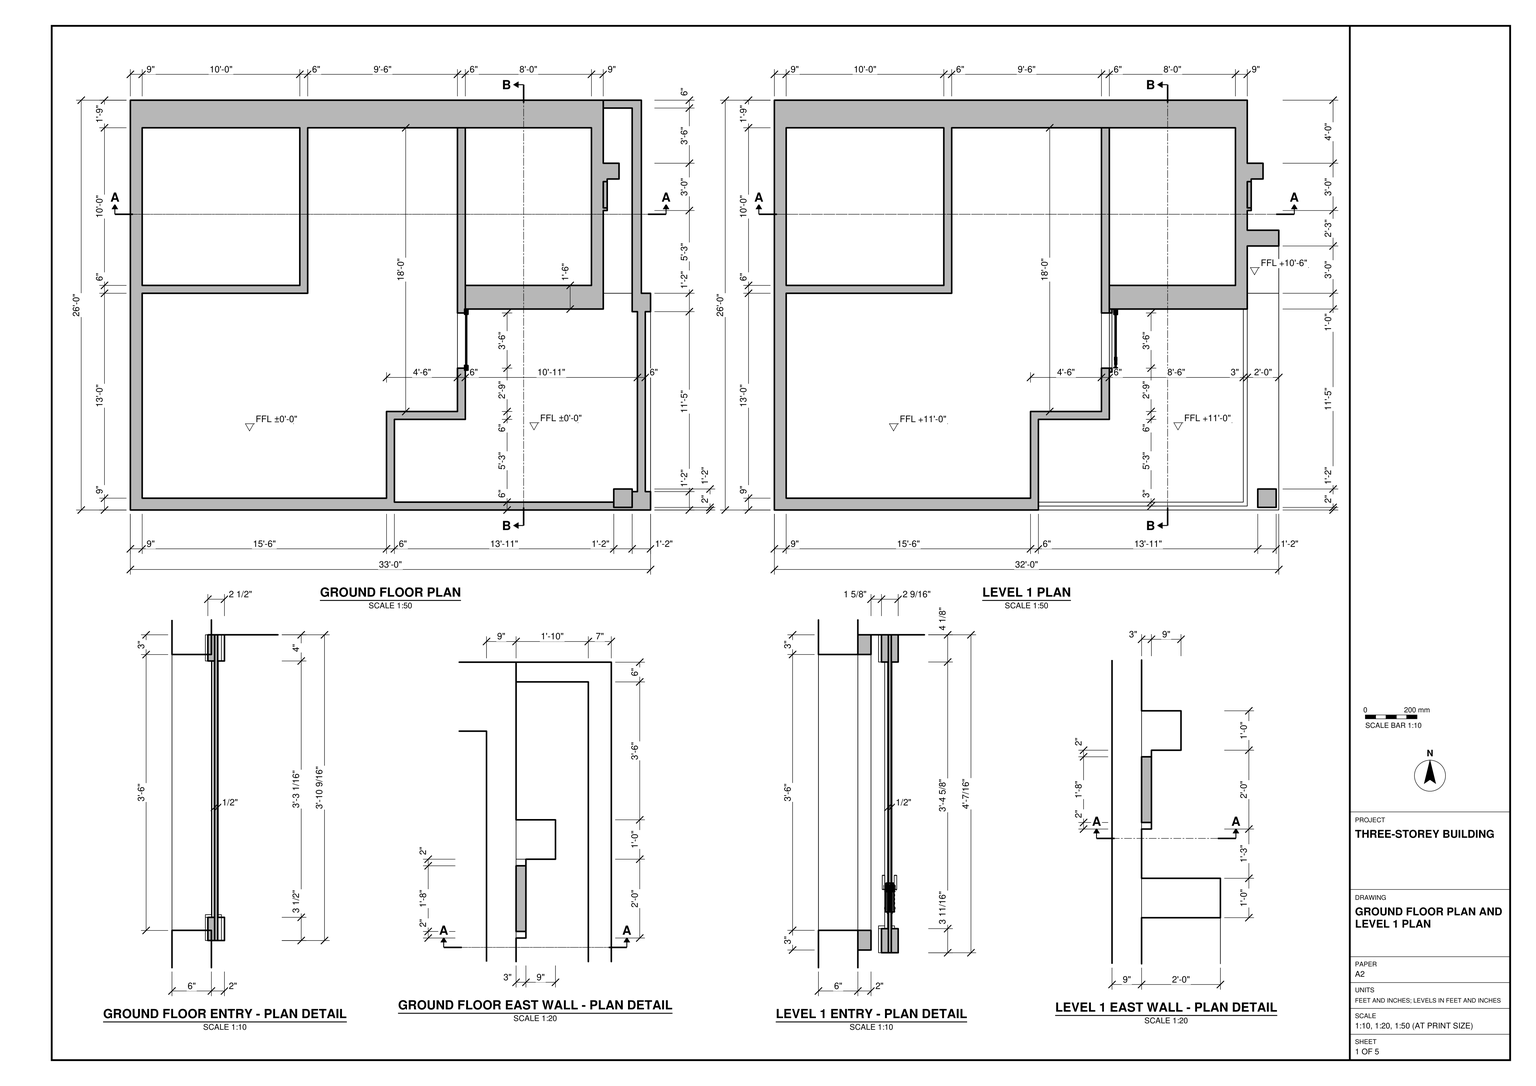
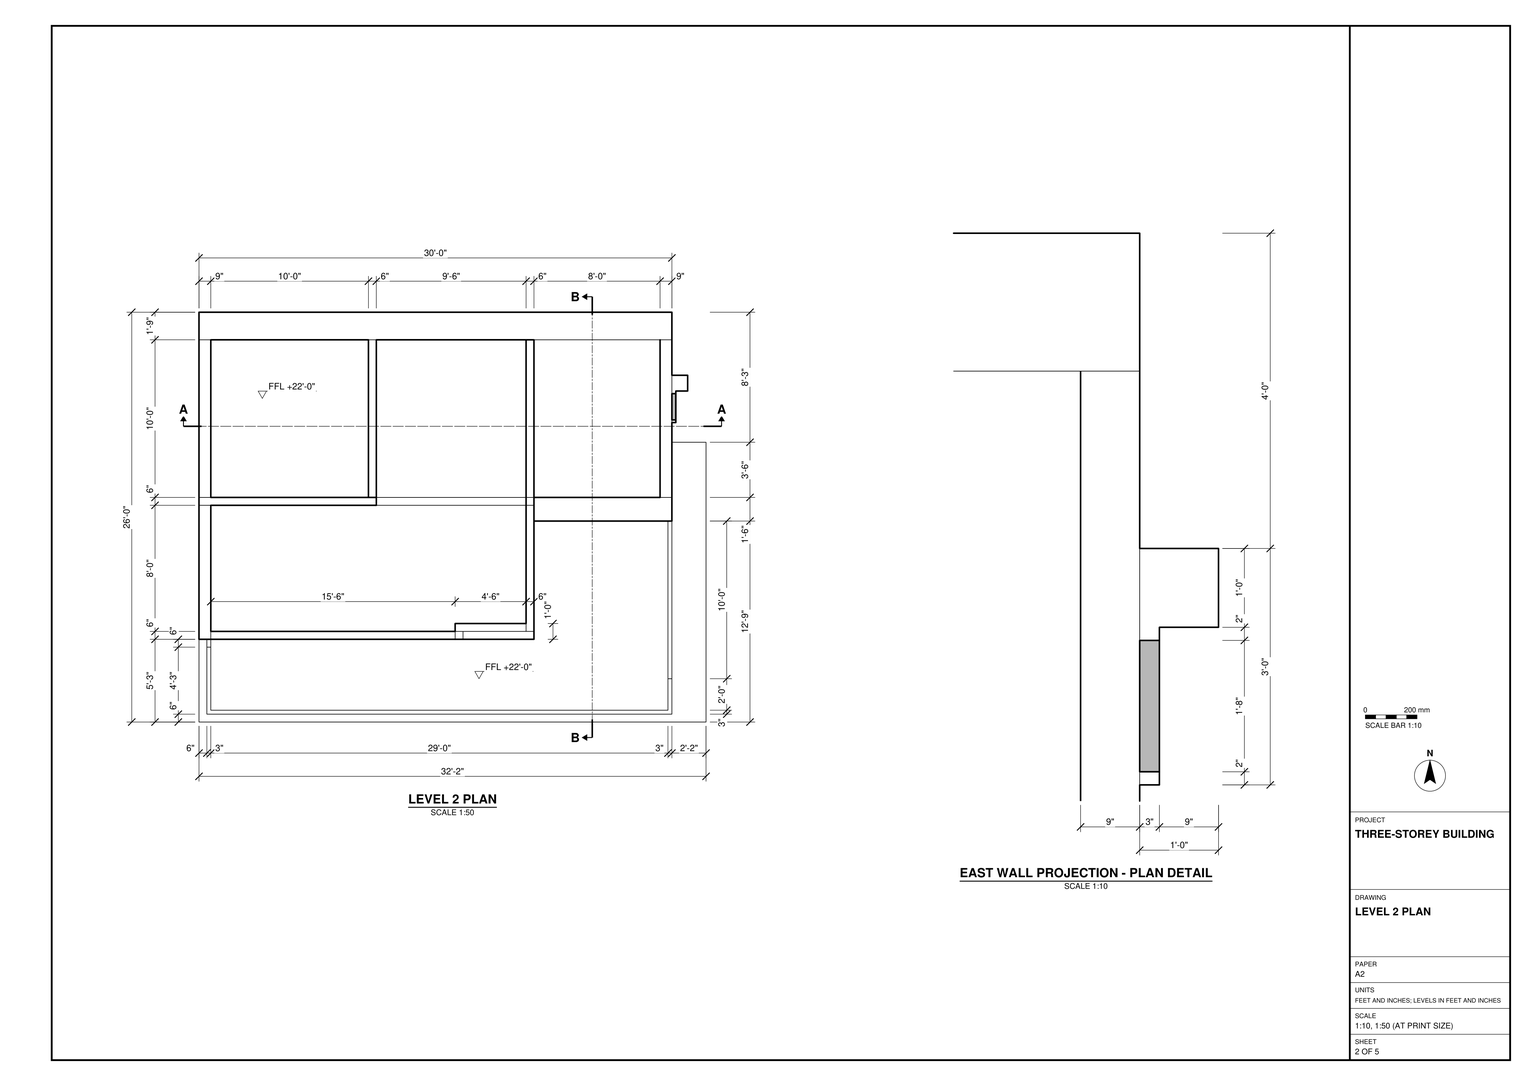
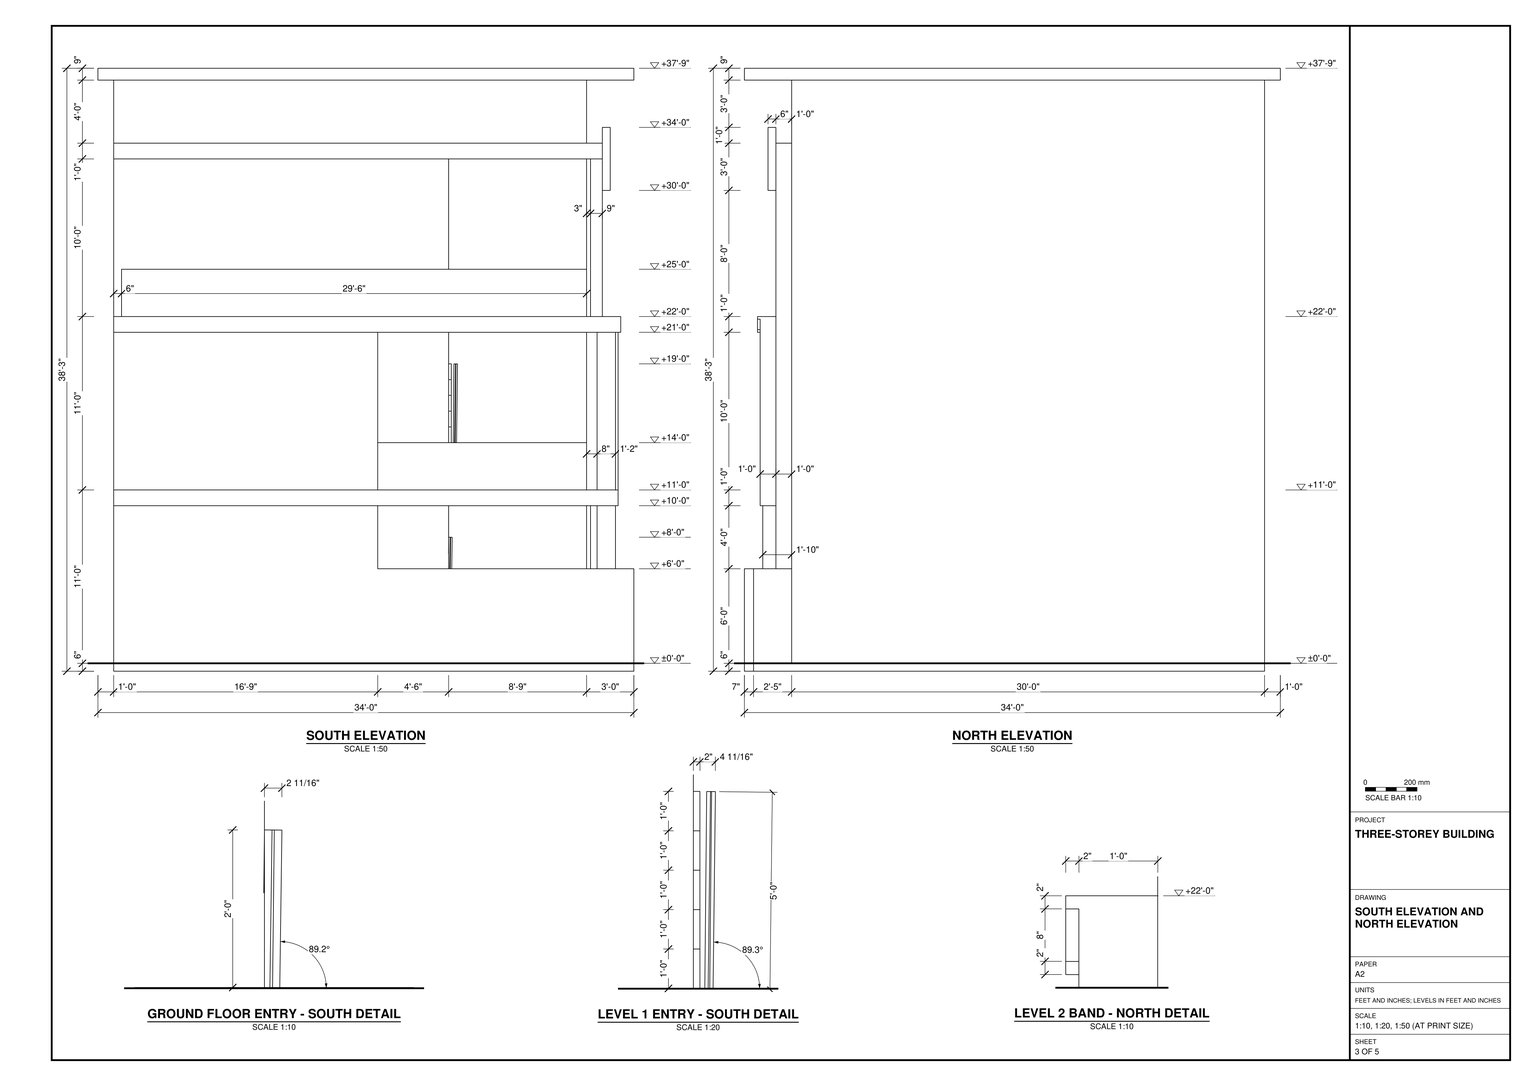
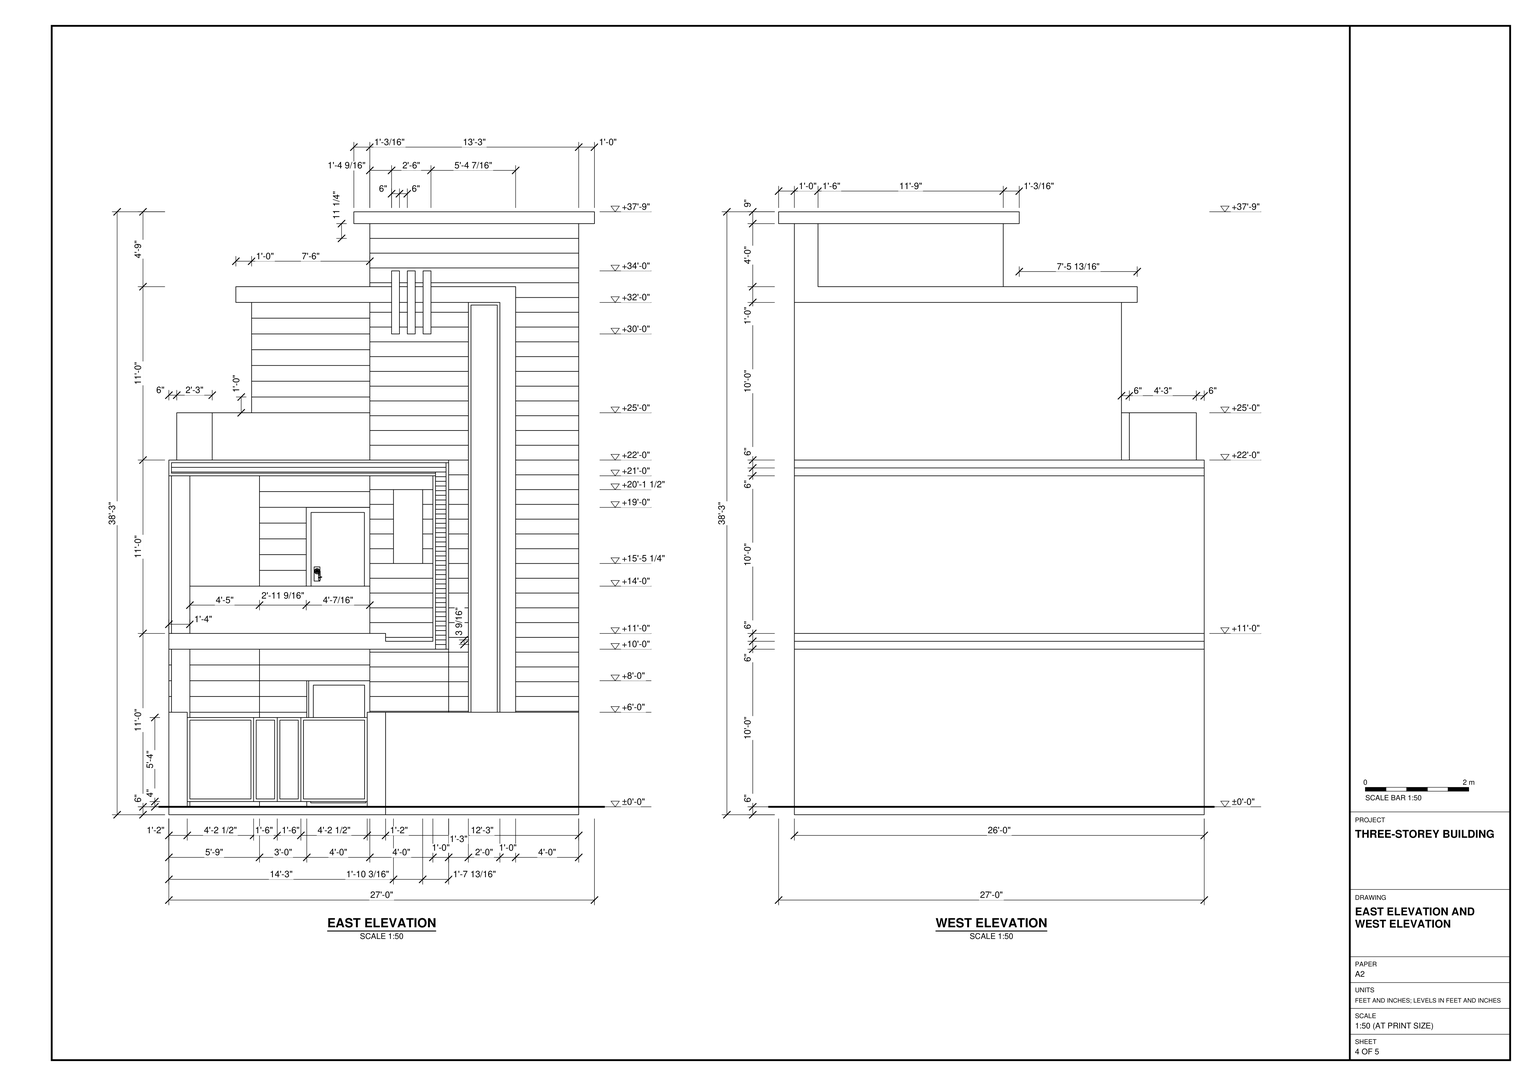
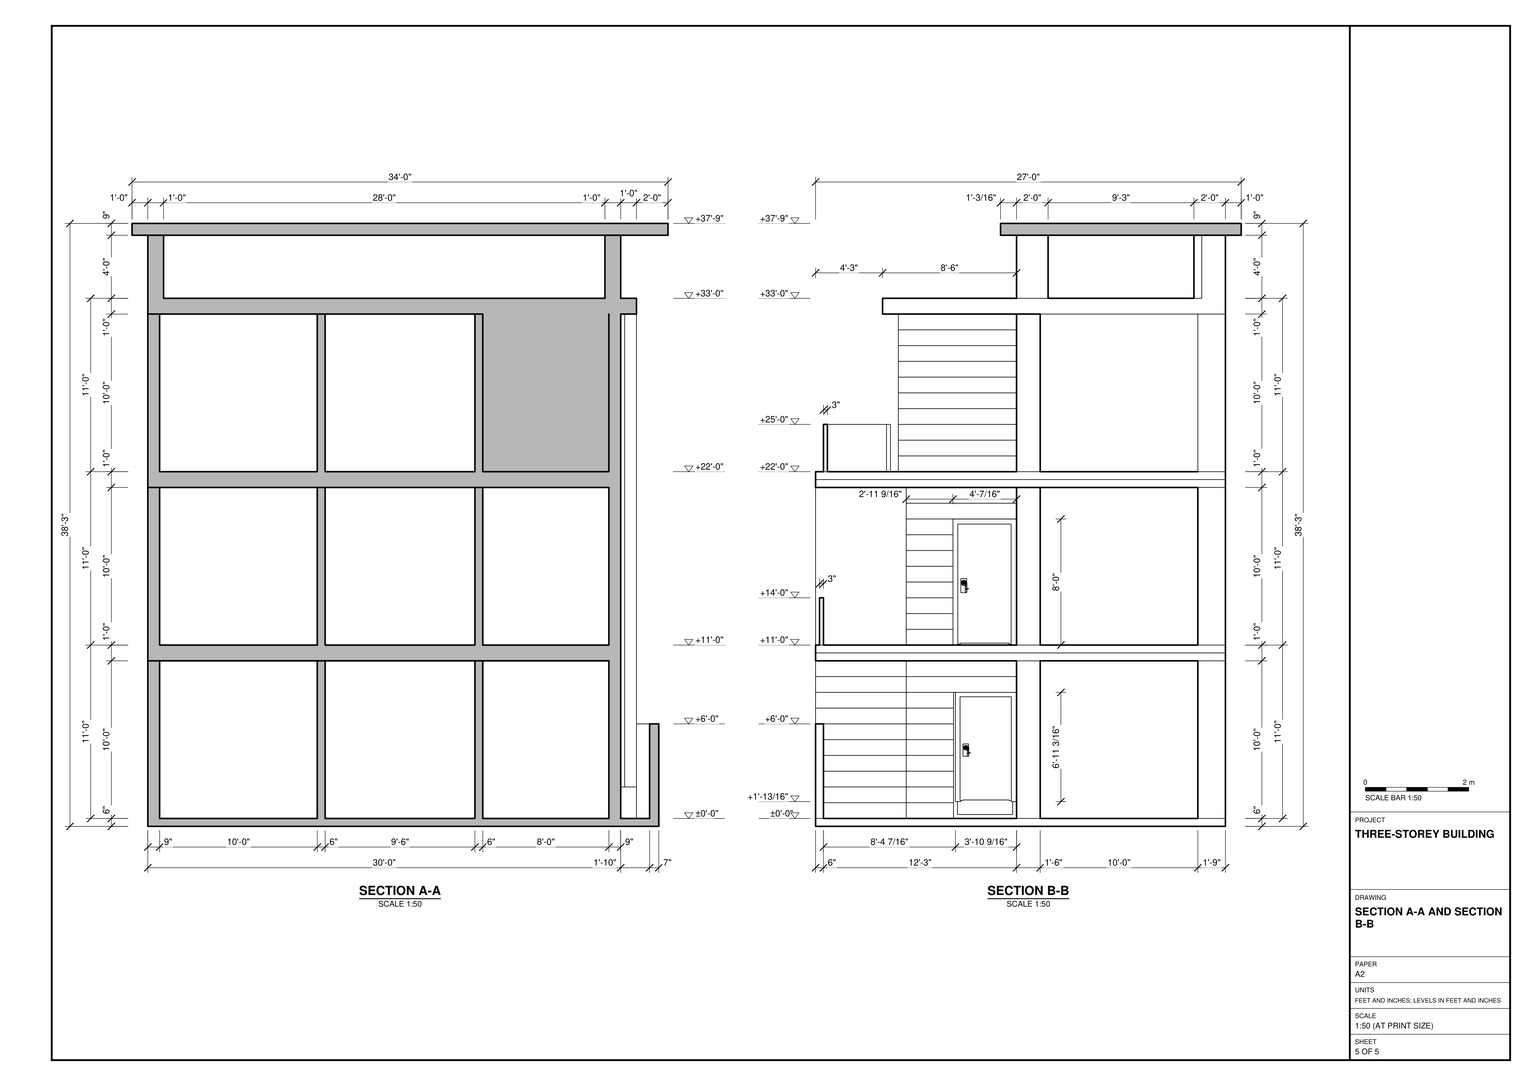
Build the three-storey building in SketchUp using task_files/diagram_01.pdf. Work in feet and inches. Set out an overall width of 34'-0" east to west, a depth of 27'-0" north to south and a height of 38'-3". Use finished floor levels of ±0'-0", +11'-0" and +22'-0". The overall height includes the slab below the ground-floor datum; the top of the flat roof is at +37'-9".

Use each floor plan to lay out the walls at their drawn thicknesses. On the lower two storeys, form the northwest and northeast bays and step the interior wall back beside the southeast entry area. Model the entry openings, frames and door leaves using the detail for the corresponding floor. Follow the east-wall details for the projections rather than carrying one profile up all three storeys. Model the floor slabs, the low walls across the open areas and the overhanging roof. On Level 2, follow the setback of the enclosed space so that the terrace extends along the south front and back into the southeast corner.

Keep walls, slabs and roof in separate groups or components, and group each furniture or joinery piece shown separately. Use components for repeated parts. Any decor or loose items shown may be represented by suitable library components. Save one SketchUp model as output_files/three_storey_building_with_recessed_entries_and_terrace.skp.

# SketchUp Ruby script. Lengths in inches.
U = 1.inch
M = Sketchup.active_model
def pt(a) = Geom::Point3d.new(a.map { |v| v * U })
def face(e, loops, mat)
  f = e.add_face(loops[0].map { |a| pt(a) })
  loops[1..].each { |l| e.add_face(l.map { |a| pt(a) }).erase! }
  f.material = f.back_material = mat if mat
  f
end
# faces: each face lists its corners as indices into pts; further lists are holes
def faces(e, pts, list, mat = nil) = list.each { |f| face(e, (f[0].is_a?(Array) ? f : [f]).map { |l| l.map { |i| pts[i] } }, mat) }
# xy, xz, yz: faces in a plane at the given z, y or x. An outline is a flat list of corners, or four numbers for a rectangle; further outlines are holes
def ring(l) = l.size == 4 ? [[l[0], l[1]], [l[2], l[1]], [l[2], l[3]], [l[0], l[3]]] : l.each_slice(2).to_a
def flat(e, list, mat, &to3) = list.each { |f| face(e, (f[0].is_a?(Array) ? f : [f]).map { |l| ring(l).map { |u, v| to3.(u, v) } }, mat) }
def xy(e, z, list, mat = nil) = flat(e, list, mat) { |x, y| [x, y, z] }
def xz(e, y, list, mat = nil) = flat(e, list, mat) { |x, z| [x, y, z] }
def yz(e, x, list, mat = nil) = flat(e, list, mat) { |y, z| [x, y, z] }
def lines(e, pts, list) = list.each { |a, b| e.add_line(pt(pts[a]), pt(pts[b])) }
# prism: a flat outline (further loops are holes) pulled along v
def prism(e, loops, v, mat = nil)
  f = face(e, loops, mat); d = Geom::Vector3d.new(v.map { |x| x * U })
  f.pushpull(f.normal.samedirection?(d) ? d.length : -d.length)
end
def box(e, o, s, mat = nil) = prism(e, [[o, [o[0] + s[0], o[1], o[2]], [o[0] + s[0], o[1] + s[1], o[2]], [o[0], o[1] + s[1], o[2]]]], [0, 0, s[2]], mat)
def at(x, y, z, deg = 0) = Geom::Transformation.translation(pt([x, y, z])) * Geom::Transformation.rotation(ORIGIN, Z_AXIS, deg.degrees)
def axes(o, x, y, z) = Geom::Transformation.new([*x, 0, *y, 0, *z, 0, *pt(o).to_a, 1])
def part(name) = M.definitions.add(name)
# library, detail: a bought-in or finely detailed component or shape, given as its bounding box
def library(name, o, s) = part(name).tap { |d| box(d.entities, o, s) }
def detail(e, o, s) = box(e.add_group.entities, o, s)
def put(e, d, t, mat = nil) = e.add_instance(d, t).tap { |i| i.material = mat if mat }
def group(e, t, mat = nil) = e.add_group.tap { |g| g.transformation = t; g.material = mat if mat }.entities
root = M.entities
M.materials.add("F02_Soft_Jade").color = [230, 255, 228]
M.materials.add("F07_Moss_Shine").color = [136, 186, 133]
M.materials.add("Fabric_Modern_3_1K").color = [166, 166, 166]
M.materials.add("Glass_Basic_01").color = [90, 97, 104]
M.materials["Glass_Basic_01"].alpha = 0.25
M.materials.add("M00_Soft_Cloud").color = [255, 255, 255]
M.materials.add("M06_Steel_Smoke").color = [86, 86, 86]
M.materials.add("M09_Shadow_Night").color = [0, 0, 0]
M.materials.add("Wood_Veneer_15_1K").color = [103, 69, 45]
c1 = library("porta+4",[0.2,-5.42,1.33],[46.55,4.72,83.21])
xy(root,-6,[[12,0,12,312,401,312,401,165,408,165,408,0]])
xy(root,0,[[21,9,207,9,207,75,261,75,261,291,147,291,147,165,21,165],[21,171,141,291],[267,171,363,291],[372,252,384,264]])
xy(root,0,[[213,6,380,6,380,16,394,16,394,14,408,14,408,151,394,151,394,165,372,165,372,153,267,153,267,69,213,69],[372,165,394,165,394,306,372,306,372,264,384,264,384,252,372,252]],"M00_Soft_Cloud")
xy(root,3,[[261,108,267,150]])
xy(root,4,[[398,14,404,151]],"F07_Moss_Shine")
xy(root,24,[[372,228,375,252]])
xy(root,26,[[372,230,375,250]],"M09_Shadow_Night")
xy(root,68,[[398,14,404,151]],"F07_Moss_Shine")
xy(root,72,[[213,0,408,0,408,14,394,14,394,2,380,2,380,6,213,6],[394,151,408,151,408,165,401,165,401,312,372,312,372,306,394,306]],"F07_Moss_Shine")
xy(root,93,[[261,108,267,150]])
xy(root,120,[[12,0,21,165],[21,0,213,0,213,69,261,69,261,75,207,75,207,9,21,9],[21,9,21,165,261,165,261,75,207,75,207,9],[261,69,267,165],[12,165,147,171],
  [147,165,261,171],[261,165,267,171],[12,171,21,291],[21,171,141,291],[141,171,147,291],
  [147,171,261,291],[261,171,267,291],[267,171,363,291]])
xy(root,120,[[213,0,213,69,267,69,267,153,372,153,372,213,396,213,396,18,378,18,378,0],[[378,0,396,18],[380,2,394,16]]],"F02_Soft_Jade")
xy(root,126,[[372,165,396,201]],"F02_Soft_Jade")
xy(root,132,[[21,9,207,9,207,75,261,75,261,291,147,291,147,165,21,165],[21,171,141,291],[267,171,363,291]])
xy(root,132,[[[213,0,396,0,396,165,372,165,372,3,213,3],[380,2,394,16]],[213,6,369,6,369,153,269,153,269,105,267,105,267,69,213,69]],"F02_Soft_Jade")
xy(root,132,[[267,105,269,153]],"F07_Moss_Shine")
xy(root,135,[[261,108,267,150],[267,108,269,150]],"F07_Moss_Shine")
xy(root,168,[[213,3,372,3,372,153,369,153,369,6,213,6]],"F02_Soft_Jade")
xy(root,225,[[261,108,267,150],[267,108,269,150]],"F07_Moss_Shine")
xy(root,228,[[267,105,269,153]],"F07_Moss_Shine")
xy(root,252,[[12,0,21,165],[21,0,213,0,213,69,261,69,261,75,207,75,207,9,21,9],[21,9,21,165,261,165,261,75,207,75,207,9],[261,69,267,165],[267,153,372,171],
  [12,165,147,171],[147,165,261,171],[261,165,267,171],[12,171,21,291],[21,171,141,291],
  [141,171,147,291],[147,171,261,291],[261,171,267,291],[267,171,363,291],[396,201,398,203]])
xy(root,252,[[[213,0,213,69,267,69,267,153,372,153,372,165,398,165,398,0],[380,2,394,16]],[372,165,398,171],[372,171,398,201]],"F02_Soft_Jade")
xy(root,254,[[396,2,398,165],[396,165,398,171],[396,171,398,203]])
xy(root,262,[[396,165,398,211],[396,211,398,213]])
xy(root,262,[[396,2,398,165]],"F02_Soft_Jade")
xy(root,264,[[21,69,207,69,207,75,261,75,261,165,21,165],[147,165,261,171],[21,171,141,291],[147,171,261,291],[267,171,363,291]])
xy(root,264,[[12,0,398,0,398,213,372,213,372,6,18,6,18,63,12,63],[21,9,369,9,369,153,267,153,267,63,21,63],[18,57,21,63]],"F02_Soft_Jade")
xy(root,300,[[18,6,372,6,372,33,369,33,369,9,21,9,21,57,18,57],[369,33,372,153]],"F02_Soft_Jade")
xy(root,360,[[384,169.54,390,175.54],[384,181.54,390,187.54],[384,193.54,390,199.54]],"M06_Steel_Smoke")
xy(root,382,[[372,230,375,250]],"M09_Shadow_Night")
xy(root,384,[[12,51,21,63],[12,63,267,63,267,69,21,69,21,165,12,165],[21,69,21,165,261,165,261,75,207,75,207,69],[207,69,261,75],[261,69,267,165],
  [267,153,372,171],[12,165,147,171],[147,165,261,171],[261,165,267,171],[12,171,21,291],
  [21,171,141,291],[141,171,147,291],[147,171,261,291],[261,171,267,291]])
xy(root,384,[[21,51,21,63,267,63,267,153,372,153,372,228,375,228,375,252,384,252,384,51]],"F02_Soft_Jade")
xy(root,396,[[24,177,360,288]])
xy(root,396,[[12,51,384,51,384,264,372,264,372,153,12,153]],"F02_Soft_Jade")
xy(root,408,[[384,169.54,390,175.54],[384,181.54,390,187.54],[384,193.54,390,199.54]],"M06_Steel_Smoke")
xy(root,444,[[12,153,24,312],[24,153,372,177],[24,177,360,288],[360,177,372,264],[360,264,372,288],
  [24,288,372,312]])
xy(root,444,[[[0,140.8,408,324],[12,153,372,312]]],"F02_Soft_Jade")
xy(root,453,[[0,140.8,408,324]],"F02_Soft_Jade")
xz(root,0,[[12,-6,408,0]])
xz(root,0,[[12,120,396,132],[12,252,398,264]],"F02_Soft_Jade")
xz(root,0,[[12,0,408,0,408,72,213,72,213,120,12,120],[12,132,213,252]],"F07_Moss_Shine")
xz(root,2,[[396,254,398,262]])
xz(root,2,[[380,0,394,72],[380,72,394,120],[380,132,394,252]],"F02_Soft_Jade")
xz(root,3,[[213,132,372,168]],"Glass_Basic_01")
xz(root,6,[[18,264,372,300]],"F02_Soft_Jade")
xz(root,6,[[213,0,380,12],[213,12,380,24],[213,24,380,36],[213,36,380,48],[213,48,380,60],
  [213,60,380,72]],"F07_Moss_Shine")
xz(root,6,[[213,132,369,168]],"Glass_Basic_01")
xz(root,9,[[21,0,207,120],[21,132,207,252]])
xz(root,9,[[21,264,369,300]],"F02_Soft_Jade")
xz(root,14,[[[394,0,408,72],[398,4,404,68]]],"F07_Moss_Shine")
xz(root,16,[[380,0,394,120],[380,132,394,252]],"F02_Soft_Jade")
xz(root,51,[[12,384,384,396]],"F02_Soft_Jade")
xz(root,57,[[18,264,21,300]],"F02_Soft_Jade")
xz(root,63,[[12,264,267,384]],"F07_Moss_Shine")
xz(root,69,[[21,264,207,384]])
xz(root,69,[[213,0,267,120],[213,132,267,252]],"F07_Moss_Shine")
xz(root,75,[[207,0,261,120],[207,132,261,252],[207,264,261,384]])
xz(root,105,[[267,132,269,144],[267,144,269,156],[267,156,269,168],[267,168,269,180],[267,180,269,192],
  [267,192,269,204],[267,204,269,216],[267,216,269,228]],"F07_Moss_Shine")
xz(root,108,[[261,3,267,93]])
xz(root,108,[[261,135,267,225],[267,135,269,225]],"F07_Moss_Shine")
xz(root,140.8,[[0,444,408,453]],"F02_Soft_Jade")
xz(root,150,[[261,3,267,93]])
xz(root,150,[[261,135,267,225],[267,135,269,225]],"F07_Moss_Shine")
xz(root,151,[[[394,0,408,72],[398,4,404,68]]],"F07_Moss_Shine")
xz(root,153,[[267,0,372,120],[267,132,269,228],[269,132,369,132,369,168,372,168,372,252,267,252,267,228,269,228],[267,264,369,264,369,300,372,300,372,384,267,384],[12,396,372,444]],"F07_Moss_Shine")
xz(root,165,[[21,0,147,120],[372,126,396,132],[21,132,147,252],[21,264,147,384]])
xz(root,165,[[401,-6,408,72]],"M00_Soft_Cloud")
xz(root,169.54,[[384,360,390,408]],"M06_Steel_Smoke")
xz(root,171,[[21,0,141,120],[267,0,363,120],[21,132,141,252],[267,132,363,252],[21,264,141,384],
  [141,264,147,384],[267,264,363,384]])
xz(root,175.54,[[384,360,390,408]],"M06_Steel_Smoke")
xz(root,177,[[24,396,360,444]])
xz(root,181.54,[[384,360,390,408]],"M06_Steel_Smoke")
xz(root,187.54,[[384,360,390,408]],"M06_Steel_Smoke")
xz(root,193.54,[[384,360,390,408]],"M06_Steel_Smoke")
xz(root,199.54,[[384,360,390,408]],"M06_Steel_Smoke")
xz(root,201,[[372,126,396,252]],"F02_Soft_Jade")
xz(root,203,[[396,252,398,254]])
xz(root,213,[[372,120,372,264,398,264,398,262,396,262,396,120]])
xz(root,228,[[372,24,375,384]])
xz(root,230,[[372,26,375,382]],"M09_Shadow_Night")
xz(root,250,[[372,26,375,382]],"M09_Shadow_Night")
xz(root,252,[[372,0,384,24],[375,24,384,384]],"F02_Soft_Jade")
xz(root,264,[[372,0,384,396]])
xz(root,288,[[24,396,360,444]])
xz(root,291,[[21,0,141,120],[147,0,261,120],[261,0,267,120],[267,0,363,120],[21,132,141,252],
  [147,132,261,252],[261,132,267,252],[267,132,363,252],[21,264,141,384],[147,264,261,384],
  [261,264,267,384]])
xz(root,306,[[372,0,394,72]],"M00_Soft_Cloud")
xz(root,312,[[12,-6,12,0,372,0,372,72,401,72,401,-6],[12,0,372,444]],"F07_Moss_Shine")
xz(root,324,[[0,444,408,453]])
yz(root,0,[[140.8,444,324,453]])
yz(root,12,[[0,-6,312,0],[0,120,312,126],[0,126,312,132],[0,252,312,258],[0,258,312,264],
  [51,384,51,396,294,396,294,444,312,444,312,384]])
yz(root,12,[[0,0,312,120],[0,132,312,252],[63,264,312,384],[153,396,294,444]],"F07_Moss_Shine")
yz(root,18,[[6,264,57,300]],"F02_Soft_Jade")
yz(root,21,[[9,0,165,120],[171,0,291,120],[9,132,165,252],[171,132,291,252],[69,264,165,384],
  [171,264,291,384]])
yz(root,21,[[9,264,54,300],[54,264,57,300]],"F02_Soft_Jade")
yz(root,24,[[177,396,288,444]])
yz(root,141,[[171,0,291,120],[171,132,291,252],[171,264,291,384]])
yz(root,147,[[165,0,291,120],[165,132,291,252],[165,264,171,384],[171,264,291,384]])
yz(root,207,[[9,0,75,120],[9,132,75,252],[69,264,75,384]])
yz(root,213,[[6,0,69,12],[6,12,69,24],[6,24,69,36],[6,36,69,48],[6,48,69,60],
  [6,60,69,72],[0,72,69,84],[0,84,69,96],[0,96,69,108],[0,108,69,120],
  [0,132,3,132,3,168,6,168,6,132,69,132,69,252,0,252]],"F07_Moss_Shine")
yz(root,261,[[[75,0,165,120],[108,3,150,93]],[165,0,171,120],[171,0,291,120],[[75,132,165,252],[108,135,150,225]],[165,132,171,252],
  [171,132,291,252],[75,264,165,384],[165,264,171,384],[171,264,291,384]])
yz(root,267,[[[105,0,153,96],[108,3,150,93]],[153,0,171,120],[171,0,291,120],[[105,132,153,228],[108,135,150,225]],[153,132,171,252],
  [171,132,291,252],[153,264,171,384],[171,264,291,384]])
yz(root,267,[[69,0,105,12],[69,12,105,24],[69,24,105,36],[69,36,105,48],[69,48,105,60],
  [69,60,105,72],[69,72,105,84],[69,84,105,96],[69,96,153,108],[69,108,153,120],
  [69,132,105,144],[69,144,105,156],[69,156,105,168],[69,168,105,180],[69,180,105,192],
  [69,192,105,204],[69,204,105,216],[69,216,105,228],[69,228,153,240],[69,240,153,252],
  [63,264,153,276],[63,276,153,288],[63,288,153,300],[63,300,153,312],[63,312,153,324],
  [63,324,153,336],[63,336,153,348],[63,348,153,360],[63,360,153,372],[63,372,153,384]],"F07_Moss_Shine")
yz(root,269,[[[105,132,153,228],[108,135,150,225]]],"F07_Moss_Shine")
yz(root,360,[[177,396,264,444],[264,396,288,444]])
yz(root,363,[[171,0,291,120],[171,132,291,252],[171,264,291,384]])
yz(root,369,[[9,264,33,300]],"F02_Soft_Jade")
yz(root,369,[[6,132,153,168],[33,264,153,300]],"Glass_Basic_01")
yz(root,372,[[252,0,264,5.25]])
yz(root,372,[[153,24,213,39],[153,39,213,50.25],[153,50.25,213,61.5],[153,61.5,213,72.75],[153,72.75,213,84],
  [153,84,213,95.25],[153,95.25,213,106.5],[153,106.5,213,117.75]],"F02_Soft_Jade")
yz(root,372,[[153,0,252,5.25],[264,0,306,5.25],[306,0,312,5.25],[153,5.25,252,16.5],[264,5.25,306,16.5],
  [306,5.25,312,16.5],[153,16.5,252,24],[264,16.5,306,27.75],[306,16.5,312,27.75],[213,24,228,27.75],
  [213,27.75,228,39],[264,27.75,306,39],[306,27.75,312,39],[213,39,228,50.25],[264,39,306,50.25],
  [306,39,312,50.25],[213,50.25,228,61.5],[264,50.25,306,61.5],[213,61.5,228,72.75],[264,61.5,306,61.5,306,72,312,72,312,72.75,264,72.75],
  [306,61.5,312,72],[213,72.75,228,84],[264,72.75,312,84],[213,84,228,95.25],[264,84,312,95.25],
  [213,95.25,228,106.5],[264,95.25,312,106.5],[213,106.5,228,117.75],[264,106.5,312,117.75],[153,117.75,213,120],
  [213,117.75,228,129],[264,117.75,312,129],[165,126,201,129],[165,129,201,129,201,140.25,153,140.25,153,132,165,132],[213,129,228,140.25],
  [264,129,312,140.25],[153,140.25,201,151.5],[213,140.25,228,151.5],[264,140.25,312,151.5],[153,151.5,201,162.75],
  [213,151.5,228,162.75],[264,151.5,312,162.75],[153,162.75,201,174],[213,162.75,228,174],[264,162.75,312,174],
  [153,174,201,185.25],[213,174,228,185.25],[264,174,312,185.25],[153,185.25,171,196.5],[193.21,185.25,201,196.5],
  [213,185.25,228,196.5],[264,185.25,312,196.5],[153,196.5,171,207.75],[193.21,196.5,201,207.75],[213,196.5,228,207.75],
  [264,196.5,312,207.75],[153,207.75,171,219],[193.21,207.75,201,219],[213,207.75,228,219],[264,207.75,312,219],
  [153,219,171,230.25],[193.21,219,201,230.25],[213,219,228,230.25],[264,219,312,230.25],[153,230.25,171,241.5],
  [193.21,230.25,201,241.5],[213,230.25,228,241.5],[264,230.25,312,241.5],[153,241.5,201,252],[213,241.5,228,252.75],
  [264,241.5,312,252.75],[213,252.75,228,264],[264,252.75,312,264],[6,264,33,300],[153,264,228,275.25],
  [264,264,312,275.25],[153,275.25,228,286.5],[264,275.25,312,286.5],[153,286.5,228,297.75],[264,286.5,312,297.75],
  [153,297.75,228,309],[264,297.75,312,309],[153,309,228,320.25],[264,309,312,320.25],[153,320.25,228,331.5],
  [264,320.25,312,331.5],[153,331.5,228,342.75],[264,331.5,312,342.75],[153,342.75,228,354],[264,342.75,312,354],
  [153,354,228,365.25],[264,354,312,365.25],[153,365.25,228,376.5],[264,365.25,312,376.5],[153,376.5,228,384],
  [264,376.5,312,387.75],[264,387.75,312,387.75,312,399,153,399,153,396,264,396],[153,399,312,410.25],[153,410.25,312,421.5],[153,421.5,312,432.75],
  [153,432.75,312,444]],"F07_Moss_Shine")
yz(root,372,[[171,185.25,193.21,241.5]],"Fabric_Modern_3_1K")
yz(root,372,[[3,132,153,168],[33,264,153,300]],"Glass_Basic_01")
yz(root,372,[[306,50.25,312,61.5]],"M00_Soft_Cloud")
yz(root,372,[[230,26,250,382]],"M09_Shadow_Night")
yz(root,375,[[[228,24,252,384],[230,26,250,382]]])
yz(root,375,[[230,26,250,382]],"Glass_Basic_01")
yz(root,380,[[6,0,6,72,2,72,2,120,16,120,16,0],[2,132,16,252]],"F02_Soft_Jade")
yz(root,380,[[2,0,6,72]],"F07_Moss_Shine")
yz(root,384,[[169.54,360,175.54,384],[181.54,360,187.54,384],[193.54,360,199.54,384],[169.54,384,175.54,396],[181.54,384,187.54,396],
  [193.54,384,199.54,396]])
yz(root,384,[[252,0,264,0,264,396,199.54,396,199.54,384,252,384],[51,384,169.54,396],[175.54,384,181.54,396],[187.54,384,193.54,396],[169.54,396,175.54,408],
  [181.54,396,187.54,408],[193.54,396,199.54,408]],"F02_Soft_Jade")
yz(root,390,[[169.54,360,175.54,408],[181.54,360,187.54,408],[193.54,360,199.54,408]],"M06_Steel_Smoke")
yz(root,394,[[14,0,16,0,16,120,2,120,2,72,14,72],[2,132,16,252]],"F02_Soft_Jade")
yz(root,394,[[2,0,14,72]],"F07_Moss_Shine")
yz(root,394,[[151,0,306,72]],"M00_Soft_Cloud")
yz(root,396,[[2,254,203,254.9]])
yz(root,396,[[0,120,203,120,203,252,201,252,201,126,165,126,165,132,0,132],[203,120,211,123.55],[211,120,213,262],[203,123.55,211,127.1],[203,127.1,211,130.65],
  [203,130.65,211,134.2],[203,134.2,211,137.75],[203,137.75,211,141.3],[203,141.3,211,144.85],[203,144.85,211,148.4],
  [203,148.4,211,151.95],[203,151.95,211,155.5],[203,155.5,211,159.05],[203,159.05,211,162.6],[203,162.6,211,166.15],
  [203,166.15,211,169.7],[203,169.7,211,173.25],[203,173.25,211,176.8],[203,176.8,211,180.35],[203,180.35,211,183.9],
  [203,183.9,211,187.45],[203,187.45,211,191],[203,191,211,194.55],[203,194.55,211,198.1],[203,198.1,211,201.65],
  [203,201.65,211,205.2],[203,205.2,211,208.75],[203,208.75,211,212.3],[203,212.3,211,215.85],[203,215.85,211,219.4],
  [203,219.4,211,222.95],[203,222.95,211,226.5],[203,226.5,211,230.05],[203,230.05,211,233.6],[203,233.6,211,237.15],
  [203,237.15,211,240.7],[203,240.7,211,244.25],[203,244.25,211,247.8],[203,247.8,211,251.35],[203,251.35,211,254.9],
  [2,254.9,211,258.45],[2,258.45,211,262]],"F02_Soft_Jade")
yz(root,398,[[0,252,203,252,203,254,2,254,2,262,213,262,213,264,0,264]],"F02_Soft_Jade")
yz(root,398,[[14,4,151,68]],"F07_Moss_Shine")
yz(root,401,[[165,-6,312,72]],"F07_Moss_Shine")
yz(root,404,[[66.5,6,80.5,66],[84.5,6,98.5,66]],"Fabric_Modern_3_1K")
yz(root,404,[[[14,4,64.5,68],[16,6,62.5,66]],[[64.5,4,82.5,68],[66.5,6,80.5,66]],[[82.5,4,100.5,68],[84.5,6,98.5,66]],[[100.5,4,151,68],[102.5,6,149,66]]],"M09_Shadow_Night")
yz(root,404,[[16,6,62.5,66],[102.5,6,149,66]],"Wood_Veneer_15_1K")
yz(root,408,[[140.8,444,324,453]],"F02_Soft_Jade")
yz(root,408,[[0,-6,165,-6,165,72,151,72,151,0,0,0],[0,0,14,72]],"F07_Moss_Shine")
p = [[147,171,0],[141,171,0],[363,291,120],[372,291,120],[147,171,132],[141,171,132],
  [363,291,252],[372,291,252],[267,69,264],[207,69,264],[372,177,387.75],[372,264,387.75],
  [372,165,387.75],[372,228,376.5],[372,230,376.5],[372,250,376.5],[372,264,376.5],[372,250,365.25],
  [372,264,365.25],[372,228,365.25],[372,230,365.25],[372,250,354],[372,264,354],[372,228,354],
  [372,230,354],[372,250,342.75],[372,264,342.75],[372,228,342.75],[372,230,342.75],[372,250,331.5],
  [372,264,331.5],[372,228,331.5],[372,230,331.5],[372,250,320.25],[372,264,320.25],[372,228,320.25],
  [372,230,320.25],[372,250,309],[372,264,309],[372,228,309],[372,230,309],[372,250,297.75],
  [372,264,297.75],[372,228,297.75],[372,230,297.75],[372,250,286.5],[372,264,286.5],[372,228,286.5],
  [372,230,286.5],[372,250,275.25],[372,264,275.25],[372,228,275.25],[372,230,275.25],[372,228,264],
  [372,230,264],[372,250,264],[372,264,264],[372,177,252.75],[372,213,252.75],[372,165,252.75],
  [372,228,252.75],[372,230,252.75],[372,250,252.75],[372,264,252.75],[372,201,241.5],[372,213,241.5],
  [372,228,241.5],[372,230,241.5],[372,250,241.5],[372,264,241.5],[372,201,230.25],[372,213,230.25],
  [372,228,230.25],[372,230,230.25],[372,250,230.25],[372,264,230.25],[372,201,219],[372,213,219],
  [372,250,219],[372,264,219],[372,228,219],[372,230,219],[372,201,207.75],[372,213,207.75],
  [372,228,207.75],[372,230,207.75],[372,250,207.75],[372,264,207.75],[372,228,196.5],[372,230,196.5],
  [372,201,196.5],[372,213,196.5],[372,250,196.5],[372,264,196.5],[372,201,185.25],[372,213,185.25],
  [372,228,185.25],[372,230,185.25],[372,250,185.25],[372,264,185.25],[372,201,174],[372,213,174],
  [372,228,174],[372,230,174],[372,250,174],[372,264,174],[372,228,162.75],[372,230,162.75],
  [372,201,162.75],[372,213,162.75],[372,250,162.75],[372,264,162.75],[372,228,151.5],[372,230,151.5],
  [372,201,151.5],[372,213,151.5],[372,250,151.5],[372,264,151.5],[372,201,140.25],[372,213,140.25],
  [372,228,140.25],[372,230,140.25],[372,250,140.25],[372,264,140.25],[372,228,129],[372,230,129],
  [372,201,129],[372,213,129],[372,250,129],[372,264,129],[372,228,117.75],[372,230,117.75],
  [372,250,117.75],[372,264,117.75],[372,228,106.5],[372,230,106.5],[372,250,106.5],[372,264,106.5],
  [372,228,95.25],[372,230,95.25],[372,250,95.25],[372,264,95.25],[372,228,84],[372,230,84],
  [372,250,84],[372,264,84],[372,228,72.75],[372,230,72.75],[372,250,72.75],[372,264,72.75],
  [372,228,61.5],[372,230,61.5],[372,250,61.5],[372,264,61.5],[372,228,50.25],[372,230,50.25],
  [372,250,50.25],[372,264,50.25],[372,228,39],[372,230,39],[372,250,39],[372,264,39],
  [372,228,27.75],[372,230,27.75],[372,250,27.75],[372,264,27.75],[372,252,16.5],[372,264,16.5],
  [372,264,0],[372,264,-6],[394,2,120],[394,2,132],[380,16,120],[380,16,132]]
lines(root,p,[[0,1],[2,3],[4,5],[6,7],[8,9],[10,11],[12,10],[13,14],[15,16],[17,18],[19,20],[21,22],
  [23,24],[25,26],[27,28],[29,30],[31,32],[33,34],[35,36],[37,38],[39,40],[41,42],[43,44],[45,46],
  [47,48],[49,50],[51,52],[53,54],[55,56],[57,58],[59,57],[60,61],[62,63],[64,65],[66,67],[68,69],
  [70,71],[72,73],[74,75],[76,77],[78,79],[80,81],[82,83],[84,85],[86,87],[88,89],[90,91],[92,93],
  [94,95],[96,97],[98,99],[100,101],[102,103],[104,105],[106,107],[108,109],[110,111],[112,113],[114,115],[116,117],
  [118,119],[120,121],[122,123],[124,125],[126,127],[128,129],[130,131],[132,133],[134,135],[136,137],[138,139],[140,141],
  [142,143],[144,145],[146,147],[148,149],[150,151],[152,153],[154,155],[156,157],[158,159],[160,161],[162,163],[164,165],
  [166,167],[168,169],[170,171],[171,172],[172,173]])
put(root,c1,at(264.24,106.25,11.48,90))
put(root,c1,axes([268.3,104.38,130.46],[0,1.04,0],[-1,0,0],[0,0,1.15383]))
